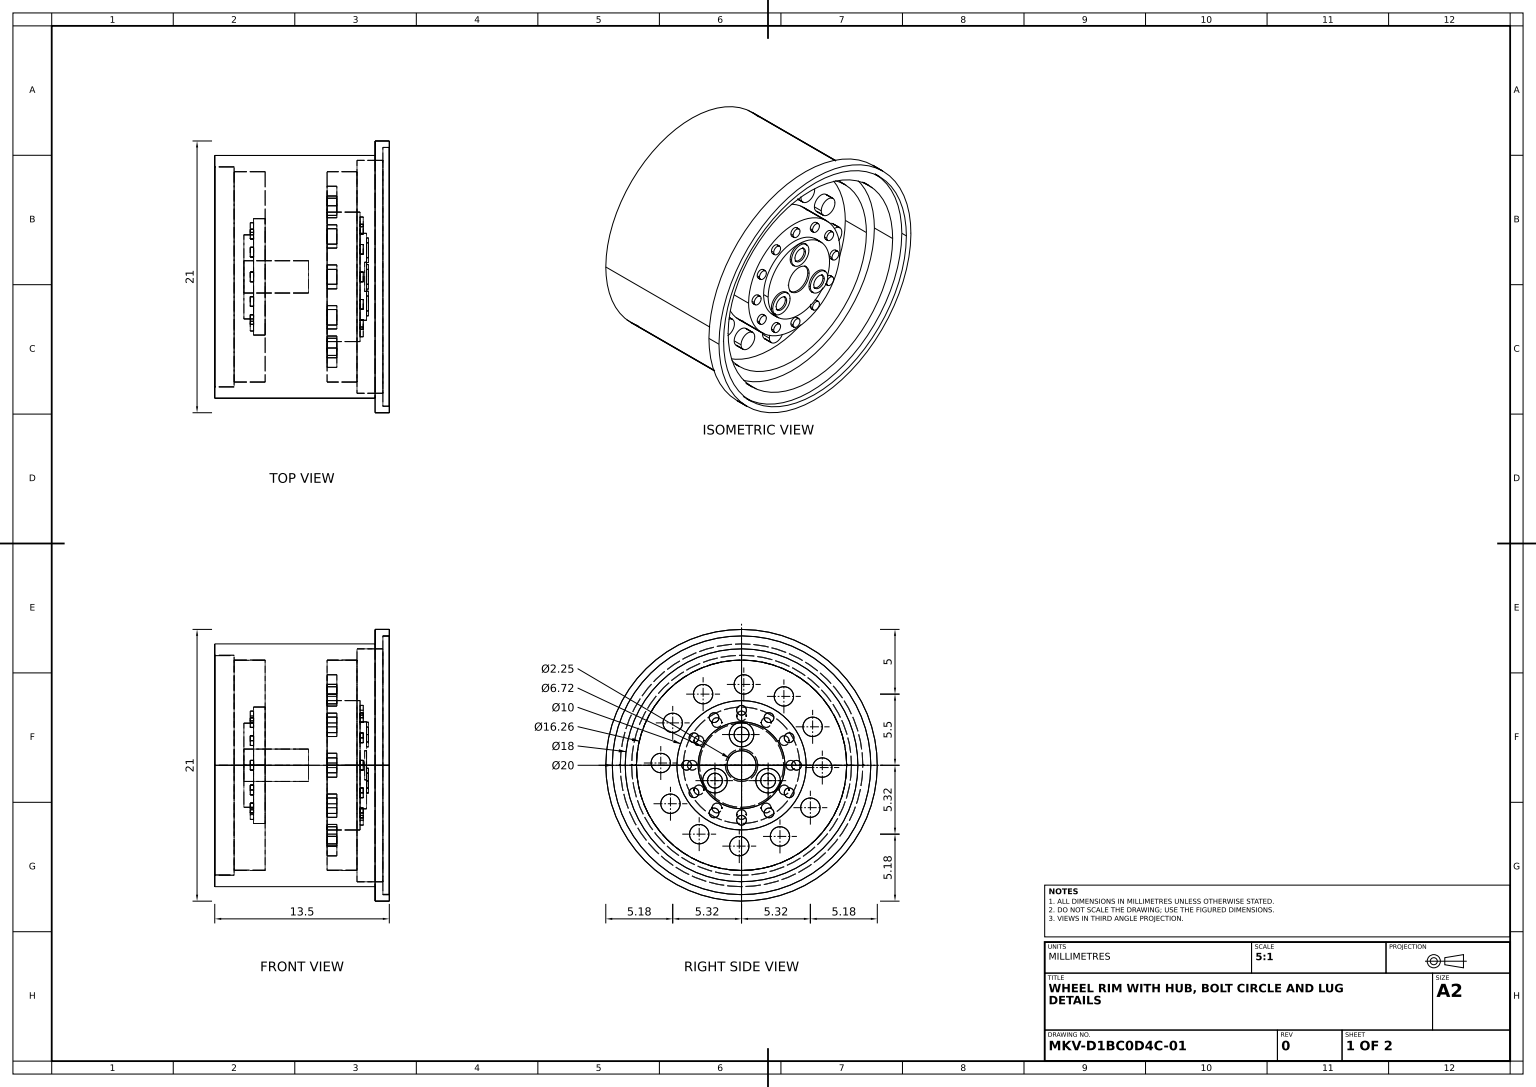
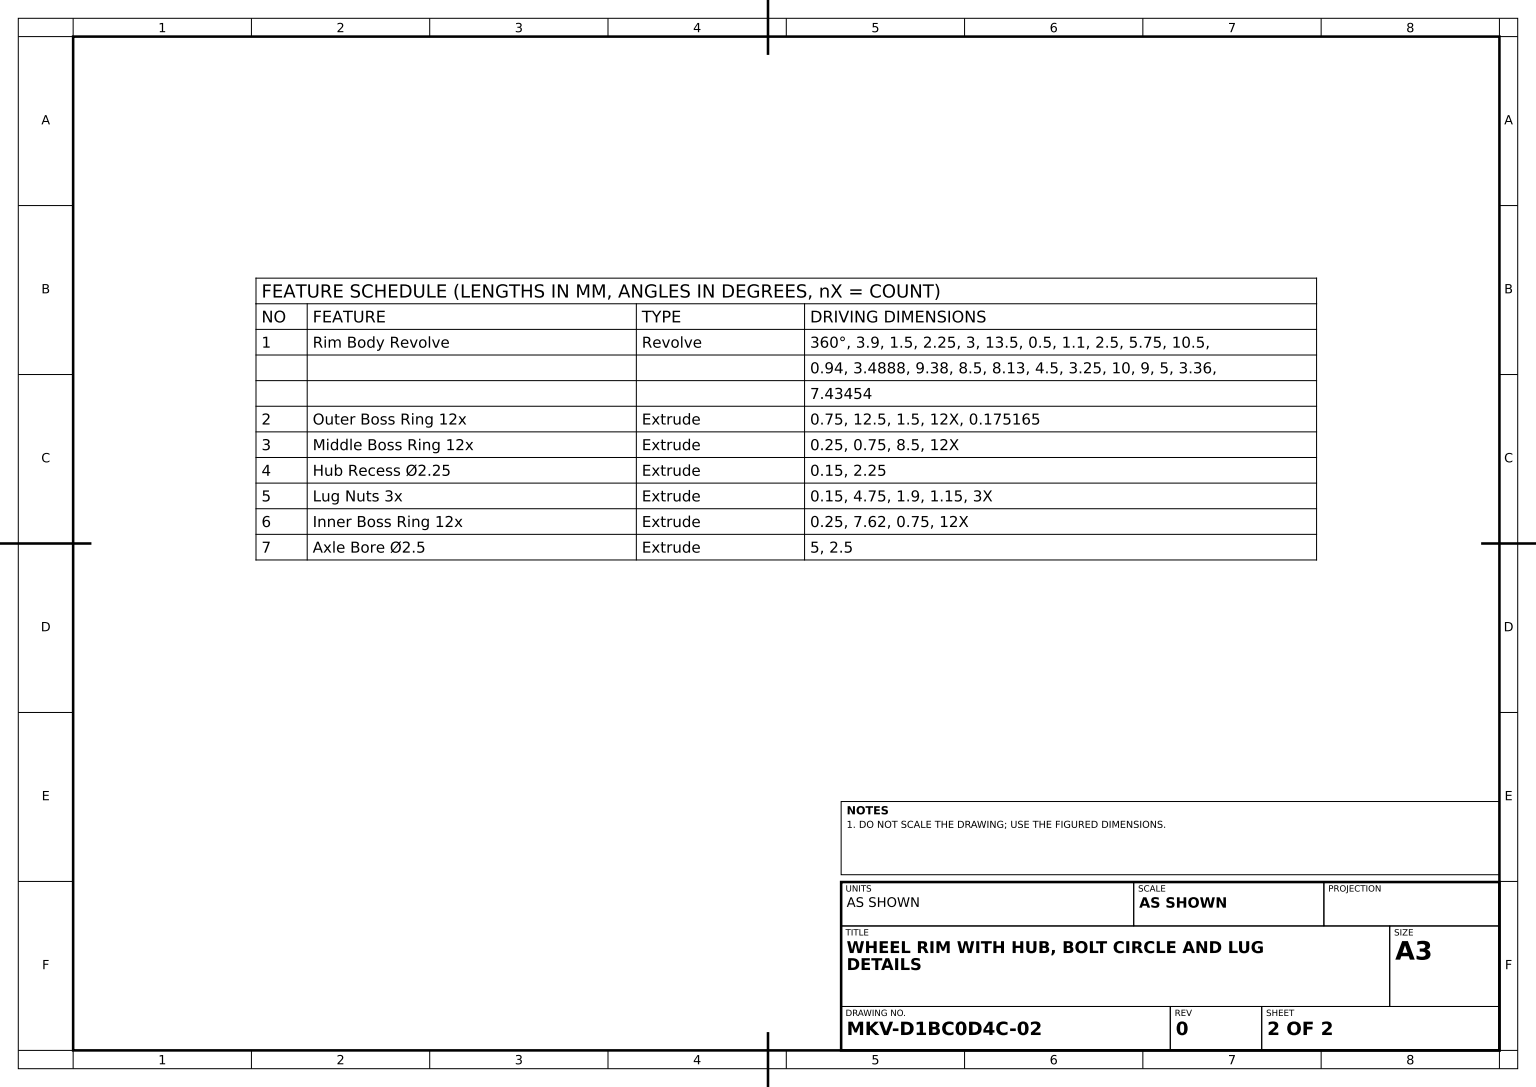
solid
v1 (1.69,6.247545,-0.925165)
v2 (0.94,6.247545,-0.925165)
e1 v1 v2 LINE
v3 (0.94,6.247545,0.574835)
e2 v2 v3 CIRCLE(AX(P(0.94,6.247545,-0.175165),D(1,0,0),D(0,0,-1)),0.75)
v4 (1.69,6.247545,0.574835)
e3 v4 v3 LINE
e4 v1 v4 CIRCLE(AX(P(1.69,6.247545,-0.175165),D(1,0,0),D(0,0,-1)),0.75)
face CYL(AX(P(1.69,6.247545,-0.175165),D(-1,0,0),D(0,0,1)),0.75) [e1 e2 -e3 -e4]
v5 (1.69,-0.175165,-6.997545)
v6 (1.69,-0.175165,-5.497545)
e5 v5 v6 CIRCLE(AX(P(1.69,-0.175165,-6.247545),D(1,0,0),D(0,0,-1)),0.75)
e6 v6 v5 CIRCLE(AX(P(1.69,-0.175165,-6.247545),D(1,0,0),D(0,0,-1)),0.75)
face PLANE(AX(P(1.69,-0.175165,-6.247545),D(1,0,0),D(0,0,-1))) [e5 e6]
v7 (-5,-3.81,0.375)
v8 (-4.75,-3.81,0.375)
e7 v7 v8 LINE
v9 (-5,-3.81,-0.375)
e8 v9 v7 CIRCLE(AX(P(-5,-3.81,0),D(-1,0,0),D(0,0,1)),0.375)
v10 (-4.75,-3.81,-0.375)
e9 v9 v10 LINE
e10 v10 v8 CIRCLE(AX(P(-4.75,-3.81,0),D(-1,0,0),D(0,0,-1)),0.375)
face CYL(AX(P(-5,-3.81,0),D(1,0,0),D(0,0,-1)),0.375) [-e7 -e8 e9 e10]
v11 (1.69,-5.498115,-2.222075)
v12 (1.69,-5.498115,-3.722075)
e11 v11 v12 CIRCLE(AX(P(1.69,-5.498115,-2.972075),D(1,0,0),D(0,0,-1)),0.75)
v13 (0.94,-5.498115,-2.222075)
e12 v11 v13 LINE
v14 (0.94,-5.498115,-3.722075)
e13 v13 v14 CIRCLE(AX(P(0.94,-5.498115,-2.972075),D(1,0,0),D(0,0,-1)),0.75)
e14 v12 v14 LINE
face CYL(AX(P(1.69,-5.498115,-2.972075),D(-1,0,0),D(0,0,1)),0.75) [-e11 e12 e13 -e14]
v15 (1.69,5.32295,-4.02547)
v16 (1.69,5.32295,-2.52547)
e15 v15 v16 CIRCLE(AX(P(1.69,5.32295,-3.27547),D(1,0,0),D(0,0,-1)),0.75)
v17 (0.94,5.32295,-4.02547)
e16 v15 v17 LINE
v18 (0.94,5.32295,-2.52547)
e17 v17 v18 CIRCLE(AX(P(0.94,5.32295,-3.27547),D(1,0,0),D(0,0,-1)),0.75)
e18 v16 v18 LINE
face CYL(AX(P(1.69,5.32295,-3.27547),D(-1,0,0),D(0,0,1)),0.75) [-e15 e16 e17 -e18]
v19 (1.69,2.972075,-6.248115)
v20 (0.94,2.972075,-6.248115)
e19 v19 v20 LINE
v21 (1.69,2.972075,-4.748115)
e20 v21 v19 CIRCLE(AX(P(1.69,2.972075,-5.498115),D(1,0,0),D(0,0,-1)),0.75)
v22 (0.94,2.972075,-4.748115)
e21 v21 v22 LINE
e22 v22 v20 CIRCLE(AX(P(0.94,2.972075,-5.498115),D(1,0,0),D(0,0,-1)),0.75)
face CYL(AX(P(1.69,2.972075,-5.498115),D(-1,0,0),D(0,0,1)),0.75) [-e19 -e20 e21 e22]
v23 (-5,1.905,-2.924557)
v24 (-5,1.905,-3.674557)
e23 v23 v24 CIRCLE(AX(P(-5,1.905,-3.299557),D(-1,0,0),D(0,0,1)),0.375)
e24 v24 v23 CIRCLE(AX(P(-5,1.905,-3.299557),D(-1,0,0),D(0,0,1)),0.375)
face PLANE(AX(P(-5,1.905,-3.299557),D(-1,0,0),D(0,0,1))) [e23 e24]
v25 (-5,-1.905,-2.924557)
v26 (-5,-1.905,-3.674557)
e25 v25 v26 CIRCLE(AX(P(-5,-1.905,-3.299557),D(-1,0,0),D(0,0,1)),0.375)
e26 v26 v25 CIRCLE(AX(P(-5,-1.905,-3.299557),D(-1,0,0),D(0,0,1)),0.375)
face PLANE(AX(P(-5,-1.905,-3.299557),D(-1,0,0),D(0,0,1))) [e25 e26]
e27 v12 v11 CIRCLE(AX(P(1.69,-5.498115,-2.972075),D(1,0,0),D(0,0,-1)),0.75)
face PLANE(AX(P(1.69,-5.498115,-2.972075),D(1,0,0),D(0,0,-1))) [e27 e11]
v27 (4.1388,-1.1875,-1.10681)
v28 (3.9888,-1.1875,-1.10681)
e28 v27 v28 LINE
v29 (4.1388,-1.1875,-3.00681)
e29 v29 v27 CIRCLE(AX(P(4.1388,-1.1875,-2.05681),D(1,0,0),D(0,0,-1)),0.95)
v30 (3.9888,-1.1875,-3.00681)
e30 v29 v30 LINE
e31 v30 v28 CIRCLE(AX(P(3.9888,-1.1875,-2.05681),D(1,0,0),D(0,0,-1)),0.95)
face CYL(AX(P(4.1388,-1.1875,-2.05681),D(-1,0,0),D(0,0,1)),0.95) [-e28 -e29 e30 e31]
v31 (-5,3.299557,1.53)
v32 (-4.75,3.299557,1.53)
e32 v31 v32 LINE
v33 (-5,3.299557,2.28)
e33 v33 v31 CIRCLE(AX(P(-5,3.299557,1.905),D(-1,0,0),D(0,0,1)),0.375)
v34 (-4.75,3.299557,2.28)
e34 v33 v34 LINE
e35 v34 v32 CIRCLE(AX(P(-4.75,3.299557,1.905),D(-1,0,0),D(0,0,-1)),0.375)
face CYL(AX(P(-5,3.299557,1.905),D(1,0,0),D(0,0,-1)),0.375) [-e32 -e33 e34 e35]
v35 (1.69,-2.972075,4.748115)
v36 (1.69,-2.972075,6.248115)
e36 v35 v36 CIRCLE(AX(P(1.69,-2.972075,5.498115),D(1,0,0),D(0,0,-1)),0.75)
e37 v36 v35 CIRCLE(AX(P(1.69,-2.972075,5.498115),D(1,0,0),D(0,0,-1)),0.75)
face PLANE(AX(P(1.69,-2.972075,5.498115),D(1,0,0),D(0,0,-1))) [e36 e37]
v37 (3.7388,-3.680608,2.5)
v38 (3.7388,-3.680608,1.75)
e38 v37 v38 CIRCLE(AX(P(3.7388,-3.680608,2.125),D(1,0,0),D(0,0,-1)),0.375)
v39 (3.4888,-3.680608,2.5)
e39 v37 v39 LINE
v40 (3.4888,-3.680608,1.75)
e40 v39 v40 CIRCLE(AX(P(3.4888,-3.680608,2.125),D(1,0,0),D(0,0,-1)),0.375)
e41 v38 v40 LINE
face CYL(AX(P(3.7388,-3.680608,2.125),D(-1,0,0),D(0,0,1)),0.375) [-e38 e39 e40 -e41]
v41 (0.94,-2.972075,4.748115)
v42 (0.94,-2.972075,6.248115)
e42 v41 v42 CIRCLE(AX(P(0.94,-2.972075,5.498115),D(1,0,0),D(0,0,-1)),0.75)
e43 v36 v42 LINE
e44 v35 v41 LINE
face CYL(AX(P(1.69,-2.972075,5.498115),D(-1,0,0),D(0,0,1)),0.75) [e42 -e43 -e36 e44]
v43 (4.1388,-1.1875,1.48181)
v44 (3.9888,-1.1875,1.48181)
e45 v43 v44 LINE
v45 (4.1388,-1.1875,2.63181)
e46 v43 v45 CIRCLE(AX(P(4.1388,-1.1875,2.05681),D(1,0,0),D(0,0,-1)),0.575)
v46 (3.9888,-1.1875,2.63181)
e47 v45 v46 LINE
e48 v46 v44 CIRCLE(AX(P(3.9888,-1.1875,2.05681),D(-1,0,0),D(0,0,-1)),0.575)
face CYL(AX(P(4.1388,-1.1875,2.05681),D(-1,0,0),D(0,0,1)),0.575) rev [-e45 e46 e47 e48]
v47 (3.7388,2.125,3.305608)
v48 (3.4888,2.125,3.305608)
e49 v47 v48 LINE
v49 (3.4888,2.125,4.055608)
e50 v48 v49 CIRCLE(AX(P(3.4888,2.125,3.680608),D(1,0,0),D(0,0,-1)),0.375)
v50 (3.7388,2.125,4.055608)
e51 v50 v49 LINE
e52 v47 v50 CIRCLE(AX(P(3.7388,2.125,3.680608),D(1,0,0),D(0,0,-1)),0.375)
face CYL(AX(P(3.7388,2.125,3.680608),D(-1,0,0),D(0,0,1)),0.375) [e49 e50 -e51 -e52]
v51 (-4.75,0,4.5)
v52 (-4.75,0,-4.5)
e53 v51 v52 CIRCLE(AX(P(-4.75,0,0),D(-1,0,0),D(0,0,1)),4.5)
v53 (-3.85,0,4.5)
e54 v53 v51 LINE
v54 (-3.85,0,-4.5)
e55 v53 v54 CIRCLE(AX(P(-3.85,0,0),D(-1,0,0),D(0,0,1)),4.5)
e56 v54 v52 LINE
face CYL(AX(P(0,0,0),D(-1,0,0),D(0,0,1)),4.5) [-e53 -e54 e55 e56]
v55 (-4.75,-3.299557,2.28)
v56 (-4.75,-3.299557,1.53)
e57 v55 v56 CIRCLE(AX(P(-4.75,-3.299557,1.905),D(-1,0,0),D(0,0,-1)),0.375)
v57 (-5,-3.299557,1.53)
e58 v57 v56 LINE
v58 (-5,-3.299557,2.28)
e59 v58 v57 CIRCLE(AX(P(-5,-3.299557,1.905),D(-1,0,0),D(0,0,1)),0.375)
e60 v58 v55 LINE
face CYL(AX(P(-5,-3.299557,1.905),D(1,0,0),D(0,0,-1)),0.375) [e57 -e58 -e59 e60]
v59 (3.7388,-4.25,-0.375)
v60 (3.4888,-4.25,-0.375)
e61 v59 v60 LINE
v61 (3.7388,-4.25,0.375)
e62 v61 v59 CIRCLE(AX(P(3.7388,-4.25,0),D(1,0,0),D(0,0,-1)),0.375)
v62 (3.4888,-4.25,0.375)
e63 v61 v62 LINE
e64 v62 v60 CIRCLE(AX(P(3.4888,-4.25,0),D(1,0,0),D(0,0,-1)),0.375)
face CYL(AX(P(3.7388,-4.25,0),D(-1,0,0),D(0,0,1)),0.375) [-e61 -e62 e63 e64]
e65 v42 v41 CIRCLE(AX(P(0.94,-2.972075,5.498115),D(1,0,0),D(0,0,-1)),0.75)
face CYL(AX(P(1.69,-2.972075,5.498115),D(-1,0,0),D(0,0,1)),0.75) [e43 e65 -e44 -e37]
v63 (3.7388,0,-3.875)
v64 (3.7388,0,-4.625)
e66 v63 v64 CIRCLE(AX(P(3.7388,0,-4.25),D(1,0,0),D(0,0,-1)),0.375)
e67 v64 v63 CIRCLE(AX(P(3.7388,0,-4.25),D(1,0,0),D(0,0,-1)),0.375)
face PLANE(AX(P(3.7388,0,-4.25),D(1,0,0),D(0,0,-1))) [e66 e67]
v65 (3.4888,0,-4.625)
v66 (3.4888,0,-3.875)
e68 v65 v66 CIRCLE(AX(P(3.4888,0,-4.25),D(1,0,0),D(0,0,-1)),0.375)
e69 v63 v66 LINE
e70 v64 v65 LINE
face CYL(AX(P(3.7388,0,-4.25),D(-1,0,0),D(0,0,1)),0.375) [e68 -e69 -e67 e70]
e71 v59 v61 CIRCLE(AX(P(3.7388,-4.25,0),D(1,0,0),D(0,0,-1)),0.375)
face PLANE(AX(P(3.7388,-4.25,0),D(1,0,0),D(0,0,-1))) [e62 e71]
v67 (-5,3.299557,-1.53)
v68 (-5,3.299557,-2.28)
e72 v67 v68 CIRCLE(AX(P(-5,3.299557,-1.905),D(-1,0,0),D(0,0,1)),0.375)
v69 (-4.75,3.299557,-1.53)
e73 v67 v69 LINE
v70 (-4.75,3.299557,-2.28)
e74 v69 v70 CIRCLE(AX(P(-4.75,3.299557,-1.905),D(-1,0,0),D(0,0,-1)),0.375)
e75 v68 v70 LINE
face CYL(AX(P(-5,3.299557,-1.905),D(1,0,0),D(0,0,-1)),0.375) [-e72 e73 e74 -e75]
v71 (-4.75,3.81,0.375)
v72 (-4.75,3.81,-0.375)
e76 v71 v72 CIRCLE(AX(P(-4.75,3.81,0),D(-1,0,0),D(0,0,-1)),0.375)
v73 (-5,3.81,-0.375)
e77 v73 v72 LINE
v74 (-5,3.81,0.375)
e78 v74 v73 CIRCLE(AX(P(-5,3.81,0),D(-1,0,0),D(0,0,1)),0.375)
e79 v74 v71 LINE
face CYL(AX(P(-5,3.81,0),D(1,0,0),D(0,0,-1)),0.375) [e76 -e77 -e78 e79]
v75 (-5,0,4.185)
v76 (-5,0,3.435)
e80 v75 v76 CIRCLE(AX(P(-5,0,3.81),D(-1,0,0),D(0,0,1)),0.375)
v77 (-4.75,0,4.185)
e81 v75 v77 LINE
v78 (-4.75,0,3.435)
e82 v77 v78 CIRCLE(AX(P(-4.75,0,3.81),D(-1,0,0),D(0,0,-1)),0.375)
e83 v76 v78 LINE
face CYL(AX(P(-5,0,3.81),D(1,0,0),D(0,0,-1)),0.375) [-e80 e81 e82 -e83]
v79 (-5,-1.905,2.924557)
v80 (-5,-1.905,3.674557)
e84 v79 v80 CIRCLE(AX(P(-5,-1.905,3.299557),D(-1,0,0),D(0,0,1)),0.375)
e85 v80 v79 CIRCLE(AX(P(-5,-1.905,3.299557),D(-1,0,0),D(0,0,1)),0.375)
face PLANE(AX(P(-5,-1.905,3.299557),D(-1,0,0),D(0,0,1))) [e84 e85]
v81 (1.69,0.175165,5.497545)
v82 (0.94,0.175165,5.497545)
e86 v81 v82 LINE
v83 (1.69,0.175165,6.997545)
e87 v83 v81 CIRCLE(AX(P(1.69,0.175165,6.247545),D(1,0,0),D(0,0,-1)),0.75)
v84 (0.94,0.175165,6.997545)
e88 v83 v84 LINE
e89 v84 v82 CIRCLE(AX(P(0.94,0.175165,6.247545),D(1,0,0),D(0,0,-1)),0.75)
face CYL(AX(P(1.69,0.175165,6.247545),D(-1,0,0),D(0,0,1)),0.75) [-e86 -e87 e88 e89]
e90 v31 v33 CIRCLE(AX(P(-5,3.299557,1.905),D(-1,0,0),D(0,0,1)),0.375)
face PLANE(AX(P(-5,3.299557,1.905),D(-1,0,0),D(0,0,1))) [e90 e33]
v85 (-0.5,0,-1.25)
v86 (-0.5,0,1.25)
e91 v85 v86 CIRCLE(AX(P(-0.5,0,0),D(-1,0,0),D(0,0,1)),1.25)
e92 v86 v85 CIRCLE(AX(P(-0.5,0,0),D(-1,0,0),D(0,0,1)),1.25)
face PLANE(AX(P(-0.5,0,0),D(-1,0,0),D(0,0,1))) [e91 e92]
v87 (3.4888,0,5)
v88 (0.94,0,5)
e93 v87 v88 LINE
v89 (0.94,0,-5)
e94 v89 v88 CIRCLE(AX(P(0.94,0,0),D(-1,0,0),D(0,0,1)),5)
v90 (3.4888,0,-5)
e95 v90 v89 LINE
e96 v90 v87 CIRCLE(AX(P(3.4888,0,0),D(-1,0,0),D(0,0,1)),5)
face CYL(AX(P(0,0,0),D(-1,0,0),D(0,0,1)),5) [e93 -e94 -e95 e96]
v91 (-5,-3.299557,-1.53)
v92 (-5,-3.299557,-2.28)
e97 v91 v92 CIRCLE(AX(P(-5,-3.299557,-1.905),D(-1,0,0),D(0,0,1)),0.375)
e98 v92 v91 CIRCLE(AX(P(-5,-3.299557,-1.905),D(-1,0,0),D(0,0,1)),0.375)
face PLANE(AX(P(-5,-3.299557,-1.905),D(-1,0,0),D(0,0,1))) [e97 e98]
v93 (3.7388,-2.125,4.055608)
v94 (3.7388,-2.125,3.305608)
e99 v93 v94 CIRCLE(AX(P(3.7388,-2.125,3.680608),D(1,0,0),D(0,0,-1)),0.375)
e100 v94 v93 CIRCLE(AX(P(3.7388,-2.125,3.680608),D(1,0,0),D(0,0,-1)),0.375)
face PLANE(AX(P(3.7388,-2.125,3.680608),D(1,0,0),D(0,0,-1))) [e99 e100]
v95 (0.94,0,-8.13)
v96 (0.94,0,8.13)
e101 v95 v96 CIRCLE(AX(P(0.94,0,0),D(-1,0,0),D(0,0,1)),8.13)
v97 (3.25,0,8.13)
e102 v97 v96 LINE
v98 (3.25,0,-8.13)
e103 v98 v97 CIRCLE(AX(P(3.25,0,0),D(-1,0,0),D(0,0,1)),8.13)
e104 v98 v95 LINE
face CYL(AX(P(0,0,0),D(-1,0,0),D(0,0,1)),8.13) rev [e101 -e102 -e103 e104]
e105 v81 v83 CIRCLE(AX(P(1.69,0.175165,6.247545),D(1,0,0),D(0,0,-1)),0.75)
face PLANE(AX(P(1.69,0.175165,6.247545),D(1,0,0),D(0,0,-1))) [e105 e87]
v99 (-7.75,0,9.38)
v100 (-7.75,0,-9.38)
e106 v99 v100 CIRCLE(AX(P(-7.75,0,0),D(-1,0,0),D(0,0,1)),9.38)
e107 v100 v99 CIRCLE(AX(P(-7.75,0,0),D(-1,0,0),D(0,0,1)),9.38)
v101 (-7.75,0,8.5)
v102 (-7.75,0,-8.5)
e108 v101 v102 CIRCLE(AX(P(-7.75,0,0),D(-1,0,0),D(0,0,1)),8.5)
e109 v102 v101 CIRCLE(AX(P(-7.75,0,0),D(-1,0,0),D(0,0,1)),8.5)
face PLANE(AX(P(-7.75,0,0),D(1,0,0),D(0,0,-1))) rev [e106 e107] [-e108 -e109]
v103 (3.9888,-1.1875,-2.63181)
v104 (3.9888,-1.1875,-1.48181)
e110 v103 v104 CIRCLE(AX(P(3.9888,-1.1875,-2.05681),D(-1,0,0),D(0,0,-1)),0.575)
v105 (4.1388,-1.1875,-1.48181)
e111 v105 v104 LINE
v106 (4.1388,-1.1875,-2.63181)
e112 v105 v106 CIRCLE(AX(P(4.1388,-1.1875,-2.05681),D(1,0,0),D(0,0,-1)),0.575)
e113 v106 v103 LINE
face CYL(AX(P(4.1388,-1.1875,-2.05681),D(-1,0,0),D(0,0,1)),0.575) rev [e110 -e111 e112 e113]
e114 v7 v9 CIRCLE(AX(P(-5,-3.81,0),D(-1,0,0),D(0,0,1)),0.375)
face PLANE(AX(P(-5,-3.81,0),D(-1,0,0),D(0,0,1))) [e8 e114]
v107 (1.69,3.27547,4.57295)
v108 (1.69,3.27547,6.07295)
e115 v107 v108 CIRCLE(AX(P(1.69,3.27547,5.32295),D(1,0,0),D(0,0,-1)),0.75)
e116 v108 v107 CIRCLE(AX(P(1.69,3.27547,5.32295),D(1,0,0),D(0,0,-1)),0.75)
face PLANE(AX(P(1.69,3.27547,5.32295),D(1,0,0),D(0,0,-1))) [e115 e116]
v109 (1.69,-6.247545,0.925165)
v110 (0.94,-6.247545,0.925165)
e117 v109 v110 LINE
v111 (1.69,-6.247545,-0.574835)
e118 v111 v109 CIRCLE(AX(P(1.69,-6.247545,0.175165),D(1,0,0),D(0,0,-1)),0.75)
v112 (0.94,-6.247545,-0.574835)
e119 v111 v112 LINE
e120 v112 v110 CIRCLE(AX(P(0.94,-6.247545,0.175165),D(1,0,0),D(0,0,-1)),0.75)
face CYL(AX(P(1.69,-6.247545,0.175165),D(-1,0,0),D(0,0,1)),0.75) [-e117 -e118 e119 e120]
v113 (-4.75,1.905,3.674557)
v114 (-4.75,1.905,2.924557)
e121 v113 v114 CIRCLE(AX(P(-4.75,1.905,3.299557),D(-1,0,0),D(0,0,-1)),0.375)
v115 (-5,1.905,2.924557)
e122 v115 v114 LINE
v116 (-5,1.905,3.674557)
e123 v116 v115 CIRCLE(AX(P(-5,1.905,3.299557),D(-1,0,0),D(0,0,1)),0.375)
e124 v116 v113 LINE
face CYL(AX(P(-5,1.905,3.299557),D(1,0,0),D(0,0,-1)),0.375) [e121 -e122 -e123 e124]
v117 (3.7388,3.680608,1.75)
v118 (3.4888,3.680608,1.75)
e125 v117 v118 LINE
v119 (3.7388,3.680608,2.5)
e126 v119 v117 CIRCLE(AX(P(3.7388,3.680608,2.125),D(1,0,0),D(0,0,-1)),0.375)
v120 (3.4888,3.680608,2.5)
e127 v119 v120 LINE
e128 v120 v118 CIRCLE(AX(P(3.4888,3.680608,2.125),D(1,0,0),D(0,0,-1)),0.375)
face CYL(AX(P(3.7388,3.680608,2.125),D(-1,0,0),D(0,0,1)),0.375) [-e125 -e126 e127 e128]
v121 (4.1388,2.375,0.95)
v122 (4.1388,2.375,-0.95)
e129 v121 v122 CIRCLE(AX(P(4.1388,2.375,0),D(1,0,0),D(0,0,-1)),0.95)
v123 (3.9888,2.375,0.95)
e130 v121 v123 LINE
v124 (3.9888,2.375,-0.95)
e131 v123 v124 CIRCLE(AX(P(3.9888,2.375,0),D(1,0,0),D(0,0,-1)),0.95)
e132 v122 v124 LINE
face CYL(AX(P(4.1388,2.375,0),D(-1,0,0),D(0,0,1)),0.95) [-e129 e130 e131 -e132]
v125 (3.7388,3.680608,-2.5)
v126 (3.4888,3.680608,-2.5)
e133 v125 v126 LINE
v127 (3.7388,3.680608,-1.75)
e134 v127 v125 CIRCLE(AX(P(3.7388,3.680608,-2.125),D(1,0,0),D(0,0,-1)),0.375)
v128 (3.4888,3.680608,-1.75)
e135 v127 v128 LINE
e136 v128 v126 CIRCLE(AX(P(3.4888,3.680608,-2.125),D(1,0,0),D(0,0,-1)),0.375)
face CYL(AX(P(3.7388,3.680608,-2.125),D(-1,0,0),D(0,0,1)),0.375) [-e133 -e134 e135 e136]
v129 (3.9888,0,1.125)
v130 (3.9888,0,-1.125)
e137 v129 v130 CIRCLE(AX(P(3.9888,0,0),D(1,0,0),D(0,0,-1)),1.125)
v131 (3.8388,0,-1.125)
e138 v131 v130 LINE
v132 (3.8388,0,1.125)
e139 v132 v131 CIRCLE(AX(P(3.8388,0,0),D(1,0,0),D(0,0,-1)),1.125)
e140 v132 v129 LINE
face CYL(AX(P(3.8388,0,0),D(1,0,0),D(0,0,-1)),1.125) rev [e137 -e138 -e139 e140]
v133 (3.7388,-2.125,-4.055608)
v134 (3.7388,-2.125,-3.305608)
e141 v133 v134 CIRCLE(AX(P(3.7388,-2.125,-3.680608),D(1,0,0),D(0,0,-1)),0.375)
e142 v134 v133 CIRCLE(AX(P(3.7388,-2.125,-3.680608),D(1,0,0),D(0,0,-1)),0.375)
face PLANE(AX(P(3.7388,-2.125,-3.680608),D(1,0,0),D(0,0,-1))) [e141 e142]
e143 v44 v46 CIRCLE(AX(P(3.9888,-1.1875,2.05681),D(-1,0,0),D(0,0,-1)),0.575)
e144 v45 v43 CIRCLE(AX(P(4.1388,-1.1875,2.05681),D(1,0,0),D(0,0,-1)),0.575)
face CYL(AX(P(4.1388,-1.1875,2.05681),D(-1,0,0),D(0,0,1)),0.575) rev [e45 e143 -e47 e144]
v135 (-4.75,1.905,-3.674557)
e145 v24 v135 LINE
v136 (-4.75,1.905,-2.924557)
e146 v135 v136 CIRCLE(AX(P(-4.75,1.905,-3.299557),D(-1,0,0),D(0,0,-1)),0.375)
e147 v23 v136 LINE
face CYL(AX(P(-5,1.905,-3.299557),D(1,0,0),D(0,0,-1)),0.375) [-e24 e145 e146 -e147]
v137 (0.94,3.27547,4.57295)
v138 (0.94,3.27547,6.07295)
e148 v137 v138 CIRCLE(AX(P(0.94,3.27547,5.32295),D(1,0,0),D(0,0,-1)),0.75)
e149 v138 v137 CIRCLE(AX(P(0.94,3.27547,5.32295),D(1,0,0),D(0,0,-1)),0.75)
v139 (0.94,-0.175165,-5.497545)
v140 (0.94,-0.175165,-6.997545)
e150 v139 v140 CIRCLE(AX(P(0.94,-0.175165,-6.247545),D(1,0,0),D(0,0,-1)),0.75)
e151 v140 v139 CIRCLE(AX(P(0.94,-0.175165,-6.247545),D(1,0,0),D(0,0,-1)),0.75)
e152 v20 v22 CIRCLE(AX(P(0.94,2.972075,-5.498115),D(1,0,0),D(0,0,-1)),0.75)
e153 v96 v95 CIRCLE(AX(P(0.94,0,0),D(-1,0,0),D(0,0,1)),8.13)
v141 (0.94,5.498115,3.722075)
v142 (0.94,5.498115,2.222075)
e154 v141 v142 CIRCLE(AX(P(0.94,5.498115,2.972075),D(1,0,0),D(0,0,-1)),0.75)
e155 v142 v141 CIRCLE(AX(P(0.94,5.498115,2.972075),D(1,0,0),D(0,0,-1)),0.75)
v143 (0.94,-5.32295,2.52547)
v144 (0.94,-5.32295,4.02547)
e156 v143 v144 CIRCLE(AX(P(0.94,-5.32295,3.27547),D(1,0,0),D(0,0,-1)),0.75)
e157 v144 v143 CIRCLE(AX(P(0.94,-5.32295,3.27547),D(1,0,0),D(0,0,-1)),0.75)
v145 (0.94,-3.27547,-6.07295)
v146 (0.94,-3.27547,-4.57295)
e158 v145 v146 CIRCLE(AX(P(0.94,-3.27547,-5.32295),D(1,0,0),D(0,0,-1)),0.75)
e159 v146 v145 CIRCLE(AX(P(0.94,-3.27547,-5.32295),D(1,0,0),D(0,0,-1)),0.75)
e160 v18 v17 CIRCLE(AX(P(0.94,5.32295,-3.27547),D(1,0,0),D(0,0,-1)),0.75)
e161 v3 v2 CIRCLE(AX(P(0.94,6.247545,-0.175165),D(1,0,0),D(0,0,-1)),0.75)
e162 v14 v13 CIRCLE(AX(P(0.94,-5.498115,-2.972075),D(1,0,0),D(0,0,-1)),0.75)
e163 v82 v84 CIRCLE(AX(P(0.94,0.175165,6.247545),D(1,0,0),D(0,0,-1)),0.75)
e164 v88 v89 CIRCLE(AX(P(0.94,0,0),D(-1,0,0),D(0,0,1)),5)
e165 v110 v112 CIRCLE(AX(P(0.94,-6.247545,0.175165),D(1,0,0),D(0,0,-1)),0.75)
face PLANE(AX(P(0.94,0,0),D(1,0,0),D(0,0,-1))) [-e148 -e149] [-e150 -e151] [-e152 -e22] [-e101 -e153] [-e154 -e155] [-e156 -e157] [-e158 -e159] [-e65 -e42] [-e160 -e17] [-e2 -e161] [-e162 -e13] [-e163 -e89] [e164 e94] [-e165 -e120]
e166 v130 v129 CIRCLE(AX(P(3.9888,0,0),D(1,0,0),D(0,0,-1)),1.125)
e167 v131 v132 CIRCLE(AX(P(3.8388,0,0),D(1,0,0),D(0,0,-1)),1.125)
face CYL(AX(P(3.8388,0,0),D(1,0,0),D(0,0,-1)),1.125) rev [e138 e166 -e140 -e167]
v147 (5.75,0,10.5)
v148 (4.65,0,10.5)
e168 v147 v148 LINE
v149 (5.75,0,-10.5)
e169 v147 v149 CIRCLE(AX(P(5.75,0,0),D(-1,0,0),D(0,0,1)),10.5)
v150 (4.65,0,-10.5)
e170 v149 v150 LINE
e171 v148 v150 CIRCLE(AX(P(4.65,0,0),D(-1,0,0),D(0,0,1)),10.5)
face CYL(AX(P(0,0,0),D(-1,0,0),D(0,0,1)),10.5) [-e168 e169 e170 -e171]
e172 v28 v30 CIRCLE(AX(P(3.9888,-1.1875,-2.05681),D(1,0,0),D(0,0,-1)),0.95)
e173 v124 v123 CIRCLE(AX(P(3.9888,2.375,0),D(1,0,0),D(0,0,-1)),0.95)
v151 (3.9888,0,-3.36)
v152 (3.9888,0,3.36)
e174 v151 v152 CIRCLE(AX(P(3.9888,0,0),D(-1,0,0),D(0,0,1)),3.36)
e175 v152 v151 CIRCLE(AX(P(3.9888,0,0),D(-1,0,0),D(0,0,1)),3.36)
v153 (3.9888,-1.1875,3.00681)
v154 (3.9888,-1.1875,1.10681)
e176 v153 v154 CIRCLE(AX(P(3.9888,-1.1875,2.05681),D(1,0,0),D(0,0,-1)),0.95)
e177 v154 v153 CIRCLE(AX(P(3.9888,-1.1875,2.05681),D(1,0,0),D(0,0,-1)),0.95)
face PLANE(AX(P(3.9888,0,0),D(1,0,0),D(0,0,-1))) [-e31 -e172] [-e166 -e137] [-e131 -e173] [-e174 -e175] [-e176 -e177]
v155 (-5,0,-3.435)
v156 (-5,0,-4.185)
e178 v155 v156 CIRCLE(AX(P(-5,0,-3.81),D(-1,0,0),D(0,0,1)),0.375)
e179 v156 v155 CIRCLE(AX(P(-5,0,-3.81),D(-1,0,0),D(0,0,1)),0.375)
face PLANE(AX(P(-5,0,-3.81),D(-1,0,0),D(0,0,1))) [e178 e179]
e180 v72 v71 CIRCLE(AX(P(-4.75,3.81,0),D(-1,0,0),D(0,0,-1)),0.375)
e181 v73 v74 CIRCLE(AX(P(-5,3.81,0),D(-1,0,0),D(0,0,1)),0.375)
face CYL(AX(P(-5,3.81,0),D(1,0,0),D(0,0,-1)),0.375) [e180 -e79 -e181 e77]
v157 (4.1388,2.375,0.575)
v158 (4.1388,2.375,-0.575)
e182 v157 v158 CIRCLE(AX(P(4.1388,2.375,0),D(1,0,0),D(0,0,-1)),0.575)
e183 v158 v157 CIRCLE(AX(P(4.1388,2.375,0),D(1,0,0),D(0,0,-1)),0.575)
e184 v122 v121 CIRCLE(AX(P(4.1388,2.375,0),D(1,0,0),D(0,0,-1)),0.95)
face PLANE(AX(P(4.1388,2.375,0),D(1,0,0),D(0,0,-1))) [-e182 -e183] [e184 e129]
v159 (3.4888,-2.125,4.055608)
e185 v93 v159 LINE
v160 (3.4888,-2.125,3.305608)
e186 v159 v160 CIRCLE(AX(P(3.4888,-2.125,3.680608),D(1,0,0),D(0,0,-1)),0.375)
e187 v94 v160 LINE
face CYL(AX(P(3.7388,-2.125,3.680608),D(-1,0,0),D(0,0,1)),0.375) [-e99 e185 e186 -e187]
v161 (-3.85,0,-8.13)
v162 (-6.25,0,-8.13)
e188 v161 v162 LINE
v163 (-6.25,0,8.13)
e189 v162 v163 CIRCLE(AX(P(-6.25,0,0),D(-1,0,0),D(0,0,1)),8.13)
v164 (-3.85,0,8.13)
e190 v164 v163 LINE
e191 v161 v164 CIRCLE(AX(P(-3.85,0,0),D(-1,0,0),D(0,0,1)),8.13)
face CYL(AX(P(0,0,0),D(-1,0,0),D(0,0,1)),8.13) rev [e188 e189 -e190 -e191]
face CYL(AX(P(4.1388,2.375,0),D(-1,0,0),D(0,0,1)),0.95) [-e130 -e184 e132 e173]
v165 (1.69,-3.27547,-6.07295)
e192 v165 v145 LINE
v166 (1.69,-3.27547,-4.57295)
e193 v166 v165 CIRCLE(AX(P(1.69,-3.27547,-5.32295),D(1,0,0),D(0,0,-1)),0.75)
e194 v166 v146 LINE
face CYL(AX(P(1.69,-3.27547,-5.32295),D(-1,0,0),D(0,0,1)),0.75) [e159 -e192 -e193 e194]
v167 (5.75,0,-10)
v168 (5.75,0,10)
e195 v167 v168 CIRCLE(AX(P(5.75,0,0),D(-1,0,0),D(0,0,1)),10)
e196 v168 v167 CIRCLE(AX(P(5.75,0,0),D(-1,0,0),D(0,0,1)),10)
e197 v149 v147 CIRCLE(AX(P(5.75,0,0),D(-1,0,0),D(0,0,1)),10.5)
face PLANE(AX(P(5.75,0,0),D(1,0,0),D(0,0,-1))) [e195 e196] [-e197 -e169]
e198 v70 v69 CIRCLE(AX(P(-4.75,3.299557,-1.905),D(-1,0,0),D(0,0,-1)),0.375)
e199 v68 v67 CIRCLE(AX(P(-5,3.299557,-1.905),D(-1,0,0),D(0,0,1)),0.375)
face CYL(AX(P(-5,3.299557,-1.905),D(1,0,0),D(0,0,-1)),0.375) [e198 -e73 -e199 e75]
v169 (5.25,0,10)
e200 v168 v169 LINE
v170 (5.25,0,-10)
e201 v169 v170 CIRCLE(AX(P(5.25,0,0),D(-1,0,0),D(0,0,1)),10)
e202 v167 v170 LINE
face CYL(AX(P(0,0,0),D(-1,0,0),D(0,0,1)),10) rev [-e196 e200 e201 -e202]
v171 (3.4888,2.125,-3.305608)
v172 (3.4888,2.125,-4.055608)
e203 v171 v172 CIRCLE(AX(P(3.4888,2.125,-3.680608),D(1,0,0),D(0,0,-1)),0.375)
v173 (3.7388,2.125,-4.055608)
e204 v173 v172 LINE
v174 (3.7388,2.125,-3.305608)
e205 v174 v173 CIRCLE(AX(P(3.7388,2.125,-3.680608),D(1,0,0),D(0,0,-1)),0.375)
e206 v174 v171 LINE
face CYL(AX(P(3.7388,2.125,-3.680608),D(-1,0,0),D(0,0,1)),0.375) [e203 -e204 -e205 e206]
e207 v104 v103 CIRCLE(AX(P(3.9888,-1.1875,-2.05681),D(-1,0,0),D(0,0,-1)),0.575)
face PLANE(AX(P(3.9888,0,0),D(1,0,0),D(0,0,-1))) [-e207 -e110]
v175 (-5.5,0,-3.25)
v176 (-5.5,0,3.25)
e208 v175 v176 CIRCLE(AX(P(-5.5,0,0),D(-1,0,0),D(0,0,1)),3.25)
e209 v176 v175 CIRCLE(AX(P(-5.5,0,0),D(-1,0,0),D(0,0,1)),3.25)
v177 (-5.5,0,-1.25)
v178 (-5.5,0,1.25)
e210 v177 v178 CIRCLE(AX(P(-5.5,0,0),D(-1,0,0),D(0,0,1)),1.25)
e211 v178 v177 CIRCLE(AX(P(-5.5,0,0),D(-1,0,0),D(0,0,1)),1.25)
face PLANE(AX(P(-5.5,0,0),D(1,0,0),D(0,0,-1))) rev [e208 e209] [-e210 -e211]
e212 v117 v119 CIRCLE(AX(P(3.7388,3.680608,2.125),D(1,0,0),D(0,0,-1)),0.375)
face PLANE(AX(P(3.7388,3.680608,2.125),D(1,0,0),D(0,0,-1))) [e126 e212]
v179 (-4.75,-3.299557,-2.28)
e213 v92 v179 LINE
v180 (-4.75,-3.299557,-1.53)
e214 v179 v180 CIRCLE(AX(P(-4.75,-3.299557,-1.905),D(-1,0,0),D(0,0,-1)),0.375)
e215 v91 v180 LINE
face CYL(AX(P(-5,-3.299557,-1.905),D(1,0,0),D(0,0,-1)),0.375) [-e98 e213 e214 -e215]
v181 (3.7388,0,4.625)
v182 (3.7388,0,3.875)
e216 v181 v182 CIRCLE(AX(P(3.7388,0,4.25),D(1,0,0),D(0,0,-1)),0.375)
e217 v182 v181 CIRCLE(AX(P(3.7388,0,4.25),D(1,0,0),D(0,0,-1)),0.375)
face PLANE(AX(P(3.7388,0,4.25),D(1,0,0),D(0,0,-1))) [e216 e217]
v183 (3.7388,4.25,-0.375)
v184 (3.7388,4.25,0.375)
e218 v183 v184 CIRCLE(AX(P(3.7388,4.25,0),D(1,0,0),D(0,0,-1)),0.375)
e219 v184 v183 CIRCLE(AX(P(3.7388,4.25,0),D(1,0,0),D(0,0,-1)),0.375)
face PLANE(AX(P(3.7388,4.25,0),D(1,0,0),D(0,0,-1))) [e218 e219]
face PLANE(AX(P(-5,3.81,0),D(-1,0,0),D(0,0,1))) [e181 e78]
e220 v54 v53 CIRCLE(AX(P(-3.85,0,0),D(-1,0,0),D(0,0,1)),4.5)
e221 v52 v51 CIRCLE(AX(P(-4.75,0,0),D(-1,0,0),D(0,0,1)),4.5)
face CYL(AX(P(0,0,0),D(-1,0,0),D(0,0,1)),4.5) [-e56 e220 e54 -e221]
v185 (-4.75,0,-3.435)
e222 v155 v185 LINE
v186 (-4.75,0,-4.185)
e223 v185 v186 CIRCLE(AX(P(-4.75,0,-3.81),D(-1,0,0),D(0,0,-1)),0.375)
e224 v156 v186 LINE
face CYL(AX(P(-5,0,-3.81),D(1,0,0),D(0,0,-1)),0.375) [-e178 e222 e223 -e224]
e225 v118 v120 CIRCLE(AX(P(3.4888,3.680608,2.125),D(1,0,0),D(0,0,-1)),0.375)
face CYL(AX(P(3.7388,3.680608,2.125),D(-1,0,0),D(0,0,1)),0.375) [-e212 e125 e225 -e127]
v187 (3.4888,0,3.36)
e226 v152 v187 LINE
v188 (3.4888,0,-3.36)
e227 v188 v187 CIRCLE(AX(P(3.4888,0,0),D(-1,0,0),D(0,0,1)),3.36)
e228 v151 v188 LINE
face CYL(AX(P(0,0,0),D(-1,0,0),D(0,0,1)),3.36) [e174 e226 -e227 -e228]
v189 (3.9888,2.375,0.575)
v190 (3.9888,2.375,-0.575)
e229 v189 v190 CIRCLE(AX(P(3.9888,2.375,0),D(-1,0,0),D(0,0,-1)),0.575)
e230 v190 v189 CIRCLE(AX(P(3.9888,2.375,0),D(-1,0,0),D(0,0,-1)),0.575)
face PLANE(AX(P(3.9888,0,0),D(1,0,0),D(0,0,-1))) [-e229 -e230]
v191 (3.7388,-3.680608,-1.75)
v192 (3.7388,-3.680608,-2.5)
e231 v191 v192 CIRCLE(AX(P(3.7388,-3.680608,-2.125),D(1,0,0),D(0,0,-1)),0.375)
e232 v192 v191 CIRCLE(AX(P(3.7388,-3.680608,-2.125),D(1,0,0),D(0,0,-1)),0.375)
face PLANE(AX(P(3.7388,-3.680608,-2.125),D(1,0,0),D(0,0,-1))) [e231 e232]
v193 (3.4888,0,3.875)
e233 v182 v193 LINE
v194 (3.4888,0,4.625)
e234 v193 v194 CIRCLE(AX(P(3.4888,0,4.25),D(1,0,0),D(0,0,-1)),0.375)
e235 v181 v194 LINE
face CYL(AX(P(3.7388,0,4.25),D(-1,0,0),D(0,0,1)),0.375) [-e217 e233 e234 -e235]
v195 (3.4888,4.25,0.375)
e236 v184 v195 LINE
v196 (3.4888,4.25,-0.375)
e237 v195 v196 CIRCLE(AX(P(3.4888,4.25,0),D(1,0,0),D(0,0,-1)),0.375)
e238 v183 v196 LINE
face CYL(AX(P(3.7388,4.25,0),D(-1,0,0),D(0,0,1)),0.375) [-e219 e236 e237 -e238]
e239 v164 v161 CIRCLE(AX(P(-3.85,0,0),D(-1,0,0),D(0,0,1)),8.13)
e240 v163 v162 CIRCLE(AX(P(-6.25,0,0),D(-1,0,0),D(0,0,1)),8.13)
face CYL(AX(P(0,0,0),D(-1,0,0),D(0,0,1)),8.13) rev [-e188 -e239 e190 e240]
e241 v5 v140 LINE
e242 v6 v139 LINE
face CYL(AX(P(1.69,-0.175165,-6.247545),D(-1,0,0),D(0,0,1)),0.75) [e150 -e241 -e6 e242]
v197 (1.69,5.498115,2.222075)
e243 v197 v142 LINE
v198 (1.69,5.498115,3.722075)
e244 v198 v197 CIRCLE(AX(P(1.69,5.498115,2.972075),D(1,0,0),D(0,0,-1)),0.75)
e245 v198 v141 LINE
face CYL(AX(P(1.69,5.498115,2.972075),D(-1,0,0),D(0,0,1)),0.75) [e154 -e243 -e244 e245]
e246 v76 v75 CIRCLE(AX(P(-5,0,3.81),D(-1,0,0),D(0,0,1)),0.375)
face PLANE(AX(P(-5,0,3.81),D(-1,0,0),D(0,0,1))) [e246 e80]
e247 v125 v127 CIRCLE(AX(P(3.7388,3.680608,-2.125),D(1,0,0),D(0,0,-1)),0.375)
face PLANE(AX(P(3.7388,3.680608,-2.125),D(1,0,0),D(0,0,-1))) [e247 e134]
e248 v106 v105 CIRCLE(AX(P(4.1388,-1.1875,-2.05681),D(1,0,0),D(0,0,-1)),0.575)
e249 v27 v29 CIRCLE(AX(P(4.1388,-1.1875,-2.05681),D(1,0,0),D(0,0,-1)),0.95)
face PLANE(AX(P(4.1388,-1.1875,-2.05681),D(1,0,0),D(0,0,-1))) [-e112 -e248] [e249 e29]
v199 (4.1388,-1.1875,1.10681)
e250 v199 v154 LINE
v200 (4.1388,-1.1875,3.00681)
e251 v200 v199 CIRCLE(AX(P(4.1388,-1.1875,2.05681),D(1,0,0),D(0,0,-1)),0.95)
e252 v200 v153 LINE
face CYL(AX(P(4.1388,-1.1875,2.05681),D(-1,0,0),D(0,0,1)),0.95) [e176 -e250 -e251 e252]
e253 v32 v34 CIRCLE(AX(P(-4.75,3.299557,1.905),D(-1,0,0),D(0,0,-1)),0.375)
face CYL(AX(P(-5,3.299557,1.905),D(1,0,0),D(0,0,-1)),0.375) [-e34 -e90 e32 e253]
e254 v187 v188 CIRCLE(AX(P(3.4888,0,0),D(-1,0,0),D(0,0,1)),3.36)
face CYL(AX(P(0,0,0),D(-1,0,0),D(0,0,1)),3.36) [e228 -e254 -e226 e175]
e255 v172 v171 CIRCLE(AX(P(3.4888,2.125,-3.680608),D(1,0,0),D(0,0,-1)),0.375)
e256 v173 v174 CIRCLE(AX(P(3.7388,2.125,-3.680608),D(1,0,0),D(0,0,-1)),0.375)
face CYL(AX(P(3.7388,2.125,-3.680608),D(-1,0,0),D(0,0,1)),0.375) [e204 e255 -e206 -e256]
e257 v86 v178 LINE
e258 v85 v177 LINE
face CYL(AX(P(-0.5,0,0),D(-1,0,0),D(0,0,1)),1.25) rev [-e92 e257 e211 -e258]
face PLANE(AX(P(3.9888,0,0),D(1,0,0),D(0,0,-1))) [-e143 -e48]
face CYL(AX(P(1.69,-5.498115,-2.972075),D(-1,0,0),D(0,0,1)),0.75) [-e27 e14 e162 -e12]
e259 v60 v62 CIRCLE(AX(P(3.4888,-4.25,0),D(1,0,0),D(0,0,-1)),0.375)
face CYL(AX(P(3.7388,-4.25,0),D(-1,0,0),D(0,0,1)),0.375) [-e63 -e71 e61 e259]
v201 (-4.75,-1.905,-2.924557)
e260 v25 v201 LINE
v202 (-4.75,-1.905,-3.674557)
e261 v201 v202 CIRCLE(AX(P(-4.75,-1.905,-3.299557),D(-1,0,0),D(0,0,-1)),0.375)
e262 v26 v202 LINE
face CYL(AX(P(-5,-1.905,-3.299557),D(1,0,0),D(0,0,-1)),0.375) [-e25 e260 e261 -e262]
e263 v66 v65 CIRCLE(AX(P(3.4888,0,-4.25),D(1,0,0),D(0,0,-1)),0.375)
face CYL(AX(P(3.7388,0,-4.25),D(-1,0,0),D(0,0,1)),0.375) [-e66 e69 e263 -e70]
e264 v8 v10 CIRCLE(AX(P(-4.75,-3.81,0),D(-1,0,0),D(0,0,-1)),0.375)
face CYL(AX(P(-5,-3.81,0),D(1,0,0),D(0,0,-1)),0.375) [e264 -e9 -e114 e7]
v203 (3.4888,-3.680608,-2.5)
v204 (3.4888,-3.680608,-1.75)
e265 v203 v204 CIRCLE(AX(P(3.4888,-3.680608,-2.125),D(1,0,0),D(0,0,-1)),0.375)
e266 v204 v203 CIRCLE(AX(P(3.4888,-3.680608,-2.125),D(1,0,0),D(0,0,-1)),0.375)
e267 v40 v39 CIRCLE(AX(P(3.4888,-3.680608,2.125),D(1,0,0),D(0,0,-1)),0.375)
v205 (3.4888,-2.125,-3.305608)
v206 (3.4888,-2.125,-4.055608)
e268 v205 v206 CIRCLE(AX(P(3.4888,-2.125,-3.680608),D(1,0,0),D(0,0,-1)),0.375)
e269 v206 v205 CIRCLE(AX(P(3.4888,-2.125,-3.680608),D(1,0,0),D(0,0,-1)),0.375)
e270 v160 v159 CIRCLE(AX(P(3.4888,-2.125,3.680608),D(1,0,0),D(0,0,-1)),0.375)
e271 v194 v193 CIRCLE(AX(P(3.4888,0,4.25),D(1,0,0),D(0,0,-1)),0.375)
e272 v126 v128 CIRCLE(AX(P(3.4888,3.680608,-2.125),D(1,0,0),D(0,0,-1)),0.375)
e273 v196 v195 CIRCLE(AX(P(3.4888,4.25,0),D(1,0,0),D(0,0,-1)),0.375)
e274 v87 v90 CIRCLE(AX(P(3.4888,0,0),D(-1,0,0),D(0,0,1)),5)
e275 v49 v48 CIRCLE(AX(P(3.4888,2.125,3.680608),D(1,0,0),D(0,0,-1)),0.375)
face PLANE(AX(P(3.4888,0,0),D(1,0,0),D(0,0,-1))) [-e265 -e266] [-e259 -e64] [-e40 -e267] [-e268 -e269] [-e186 -e270] [e227 e254] [-e234 -e271] [-e272 -e136] [-e237 -e273] [-e263 -e68] [-e255 -e203] [-e96 -e274] [-e128 -e225] [-e275 -e50]
e276 v165 v166 CIRCLE(AX(P(1.69,-3.27547,-5.32295),D(1,0,0),D(0,0,-1)),0.75)
face PLANE(AX(P(1.69,-3.27547,-5.32295),D(1,0,0),D(0,0,-1))) [e276 e193]
v207 (4.65,0,9.38)
v208 (4.65,0,-9.38)
e277 v207 v208 CIRCLE(AX(P(4.65,0,0),D(-1,0,0),D(0,0,1)),9.38)
e278 v208 v207 CIRCLE(AX(P(4.65,0,0),D(-1,0,0),D(0,0,1)),9.38)
e279 v150 v148 CIRCLE(AX(P(4.65,0,0),D(-1,0,0),D(0,0,1)),10.5)
face PLANE(AX(P(4.65,0,0),D(-1,0,0),D(0,0,1))) [-e277 -e278] [e171 e279]
e280 v97 v98 CIRCLE(AX(P(3.25,0,0),D(-1,0,0),D(0,0,1)),8.13)
face CYL(AX(P(0,0,0),D(-1,0,0),D(0,0,1)),8.13) rev [e102 e153 -e104 -e280]
face PLANE(AX(P(3.8388,0,0),D(1,0,0),D(0,0,-1))) [e139 e167]
v209 (5.25,0,9)
v210 (3.25,0,9)
e281 v209 v210 LINE
v211 (3.25,0,-9)
e282 v210 v211 CIRCLE(AX(P(3.25,0,0),D(-1,0,0),D(0,0,1)),9)
v212 (5.25,0,-9)
e283 v212 v211 LINE
e284 v209 v212 CIRCLE(AX(P(5.25,0,0),D(-1,0,0),D(0,0,1)),9)
face CYL(AX(P(0,0,0),D(-1,0,0),D(0,0,1)),9) rev [e281 e282 -e283 -e284]
v213 (-4.75,-1.905,3.674557)
e285 v80 v213 LINE
v214 (-4.75,-1.905,2.924557)
e286 v213 v214 CIRCLE(AX(P(-4.75,-1.905,3.299557),D(-1,0,0),D(0,0,-1)),0.375)
e287 v79 v214 LINE
face CYL(AX(P(-5,-1.905,3.299557),D(1,0,0),D(0,0,-1)),0.375) [e285 e286 -e287 -e85]
e288 v115 v116 CIRCLE(AX(P(-5,1.905,3.299557),D(-1,0,0),D(0,0,1)),0.375)
face PLANE(AX(P(-5,1.905,3.299557),D(-1,0,0),D(0,0,1))) [e123 e288]
e289 v108 v138 LINE
e290 v107 v137 LINE
face CYL(AX(P(1.69,3.27547,5.32295),D(-1,0,0),D(0,0,1)),0.75) [e289 e149 -e290 -e116]
e291 v19 v21 CIRCLE(AX(P(1.69,2.972075,-5.498115),D(1,0,0),D(0,0,-1)),0.75)
face PLANE(AX(P(1.69,2.972075,-5.498115),D(1,0,0),D(0,0,-1))) [e20 e291]
e292 v170 v169 CIRCLE(AX(P(5.25,0,0),D(-1,0,0),D(0,0,1)),10)
face CYL(AX(P(0,0,0),D(-1,0,0),D(0,0,1)),10) rev [e202 e292 -e200 -e195]
e293 v199 v200 CIRCLE(AX(P(4.1388,-1.1875,2.05681),D(1,0,0),D(0,0,-1)),0.95)
face CYL(AX(P(4.1388,-1.1875,2.05681),D(-1,0,0),D(0,0,1)),0.95) [e177 -e252 -e293 e250]
face CYL(AX(P(1.69,-3.27547,-5.32295),D(-1,0,0),D(0,0,1)),0.75) [e192 e158 -e194 -e276]
v215 (-4.75,0,3.25)
v216 (-4.75,0,-3.25)
e294 v215 v216 CIRCLE(AX(P(-4.75,0,0),D(-1,0,0),D(0,0,1)),3.25)
e295 v216 v175 LINE
e296 v215 v176 LINE
face CYL(AX(P(0,0,0),D(-1,0,0),D(0,0,1)),3.25) [e294 e295 -e209 -e296]
face PLANE(AX(P(-3.85,0,0),D(1,0,0),D(0,0,-1))) rev [-e55 -e220] [e239 e191]
e297 v57 v58 CIRCLE(AX(P(-5,-3.299557,1.905),D(-1,0,0),D(0,0,1)),0.375)
e298 v56 v55 CIRCLE(AX(P(-4.75,-3.299557,1.905),D(-1,0,0),D(0,0,-1)),0.375)
face CYL(AX(P(-5,-3.299557,1.905),D(1,0,0),D(0,0,-1)),0.375) [-e297 e58 e298 -e60]
face CYL(AX(P(1.69,3.27547,5.32295),D(-1,0,0),D(0,0,1)),0.75) [e290 e148 -e289 -e115]
face PLANE(AX(P(3.7388,2.125,-3.680608),D(1,0,0),D(0,0,-1))) [e256 e205]
face CYL(AX(P(3.7388,0,4.25),D(-1,0,0),D(0,0,1)),0.375) [-e216 e235 e271 -e233]
e299 v212 v209 CIRCLE(AX(P(5.25,0,0),D(-1,0,0),D(0,0,1)),9)
face PLANE(AX(P(5.25,0,0),D(1,0,0),D(0,0,-1))) [e299 e284] [-e292 -e201]
e300 v114 v113 CIRCLE(AX(P(-4.75,1.905,3.299557),D(-1,0,0),D(0,0,-1)),0.375)
face CYL(AX(P(-5,1.905,3.299557),D(1,0,0),D(0,0,-1)),0.375) [-e124 -e288 e122 e300]
v217 (1.69,-5.32295,2.52547)
v218 (1.69,-5.32295,4.02547)
e301 v217 v218 CIRCLE(AX(P(1.69,-5.32295,3.27547),D(1,0,0),D(0,0,-1)),0.75)
e302 v218 v217 CIRCLE(AX(P(1.69,-5.32295,3.27547),D(1,0,0),D(0,0,-1)),0.75)
face PLANE(AX(P(1.69,-5.32295,3.27547),D(1,0,0),D(0,0,-1))) [e301 e302]
e303 v217 v143 LINE
e304 v218 v144 LINE
face CYL(AX(P(1.69,-5.32295,3.27547),D(-1,0,0),D(0,0,1)),0.75) [e157 -e303 -e302 e304]
e305 v16 v15 CIRCLE(AX(P(1.69,5.32295,-3.27547),D(1,0,0),D(0,0,-1)),0.75)
face CYL(AX(P(1.69,5.32295,-3.27547),D(-1,0,0),D(0,0,1)),0.75) [-e305 e18 e160 -e16]
e306 v4 v1 CIRCLE(AX(P(1.69,6.247545,-0.175165),D(1,0,0),D(0,0,-1)),0.75)
face CYL(AX(P(1.69,6.247545,-0.175165),D(-1,0,0),D(0,0,1)),0.75) [e161 -e1 -e306 e3]
face CYL(AX(P(4.1388,-1.1875,-2.05681),D(-1,0,0),D(0,0,1)),0.95) [-e249 e28 e172 -e30]
e307 v192 v203 LINE
e308 v191 v204 LINE
face CYL(AX(P(3.7388,-3.680608,-2.125),D(-1,0,0),D(0,0,1)),0.375) [-e232 e307 e265 -e308]
e309 v38 v37 CIRCLE(AX(P(3.7388,-3.680608,2.125),D(1,0,0),D(0,0,-1)),0.375)
face CYL(AX(P(3.7388,-3.680608,2.125),D(-1,0,0),D(0,0,1)),0.375) [-e309 e41 e267 -e39]
face PLANE(AX(P(1.69,5.32295,-3.27547),D(1,0,0),D(0,0,-1))) [e15 e305]
e310 v133 v206 LINE
e311 v134 v205 LINE
face CYL(AX(P(3.7388,-2.125,-3.680608),D(-1,0,0),D(0,0,1)),0.375) [-e141 e310 e269 -e311]
face CYL(AX(P(3.7388,-2.125,-3.680608),D(-1,0,0),D(0,0,1)),0.375) [e268 -e310 -e142 e311]
face CYL(AX(P(1.69,-0.175165,-6.247545),D(-1,0,0),D(0,0,1)),0.75) [-e242 -e5 e241 e151]
face CYL(AX(P(-0.5,0,0),D(-1,0,0),D(0,0,1)),1.25) rev [-e257 -e91 e258 e210]
v219 (-6.25,0,-8.5)
e312 v219 v102 LINE
v220 (-6.25,0,8.5)
e313 v220 v219 CIRCLE(AX(P(-6.25,0,0),D(-1,0,0),D(0,0,1)),8.5)
e314 v220 v101 LINE
face CYL(AX(P(0,0,0),D(-1,0,0),D(0,0,1)),8.5) rev [-e312 -e313 e314 e108]
face CYL(AX(P(3.7388,3.680608,-2.125),D(-1,0,0),D(0,0,1)),0.375) [e133 e272 -e135 -e247]
face PLANE(AX(P(4.1388,-1.1875,2.05681),D(1,0,0),D(0,0,-1))) [-e46 -e144] [e251 e293]
e315 v216 v215 CIRCLE(AX(P(-4.75,0,0),D(-1,0,0),D(0,0,1)),3.25)
face CYL(AX(P(0,0,0),D(-1,0,0),D(0,0,1)),3.25) [-e208 -e295 e315 e296]
face CYL(AX(P(0,0,0),D(-1,0,0),D(0,0,1)),5) [e95 -e164 -e93 e274]
e316 v50 v47 CIRCLE(AX(P(3.7388,2.125,3.680608),D(1,0,0),D(0,0,-1)),0.375)
face PLANE(AX(P(3.7388,2.125,3.680608),D(1,0,0),D(0,0,-1))) [e52 e316]
face CYL(AX(P(3.7388,-3.680608,-2.125),D(-1,0,0),D(0,0,1)),0.375) [-e231 e308 e266 -e307]
e317 v78 v77 CIRCLE(AX(P(-4.75,0,3.81),D(-1,0,0),D(0,0,-1)),0.375)
face CYL(AX(P(-5,0,3.81),D(1,0,0),D(0,0,-1)),0.375) [e83 e317 -e81 -e246]
face PLANE(AX(P(-5,3.299557,-1.905),D(-1,0,0),D(0,0,1))) [e72 e199]
e318 v214 v213 CIRCLE(AX(P(-4.75,-1.905,3.299557),D(-1,0,0),D(0,0,-1)),0.375)
face CYL(AX(P(-5,-1.905,3.299557),D(1,0,0),D(0,0,-1)),0.375) [-e285 -e84 e287 e318]
e319 v186 v185 CIRCLE(AX(P(-4.75,0,-3.81),D(-1,0,0),D(0,0,-1)),0.375)
face CYL(AX(P(-5,0,-3.81),D(1,0,0),D(0,0,-1)),0.375) [e224 e319 -e222 -e179]
face PLANE(AX(P(1.69,6.247545,-0.175165),D(1,0,0),D(0,0,-1))) [e306 e4]
e320 v158 v190 LINE
e321 v157 v189 LINE
face CYL(AX(P(4.1388,2.375,0),D(-1,0,0),D(0,0,1)),0.575) rev [e182 e320 e230 -e321]
e322 v136 v135 CIRCLE(AX(P(-4.75,1.905,-3.299557),D(-1,0,0),D(0,0,-1)),0.375)
e323 v180 v179 CIRCLE(AX(P(-4.75,-3.299557,-1.905),D(-1,0,0),D(0,0,-1)),0.375)
e324 v202 v201 CIRCLE(AX(P(-4.75,-1.905,-3.299557),D(-1,0,0),D(0,0,-1)),0.375)
face PLANE(AX(P(-4.75,0,0),D(1,0,0),D(0,0,-1))) rev [-e322 -e146] [-e57 -e298] [-e121 -e300] [-e214 -e323] [-e294 -e315] [-e35 -e253] [-e10 -e264] [e221 e53] [-e82 -e317] [-e223 -e319] [-e76 -e180] [-e286 -e318] [-e261 -e324] [-e74 -e198]
face CYL(AX(P(4.1388,-1.1875,-2.05681),D(-1,0,0),D(0,0,1)),0.575) rev [-e113 e248 e111 e207]
face CYL(AX(P(3.7388,4.25,0),D(-1,0,0),D(0,0,1)),0.375) [e273 -e236 -e218 e238]
face PLANE(AX(P(3.7388,-3.680608,2.125),D(1,0,0),D(0,0,-1))) [e38 e309]
face CYL(AX(P(-5,-1.905,-3.299557),D(1,0,0),D(0,0,-1)),0.375) [-e26 e262 e324 -e260]
e325 v219 v220 CIRCLE(AX(P(-6.25,0,0),D(-1,0,0),D(0,0,1)),8.5)
face PLANE(AX(P(-6.25,0,0),D(1,0,0),D(0,0,-1))) rev [-e240 -e189] [e313 e325]
face CYL(AX(P(1.69,2.972075,-5.498115),D(-1,0,0),D(0,0,1)),0.75) [e152 -e21 -e291 e19]
e326 v109 v111 CIRCLE(AX(P(1.69,-6.247545,0.175165),D(1,0,0),D(0,0,-1)),0.75)
face CYL(AX(P(1.69,-6.247545,0.175165),D(-1,0,0),D(0,0,1)),0.75) [e165 -e119 -e326 e117]
e327 v208 v100 LINE
e328 v207 v99 LINE
face CYL(AX(P(0,0,0),D(-1,0,0),D(0,0,1)),9.38) [e327 -e106 -e328 e277]
face CYL(AX(P(-5,-3.299557,-1.905),D(1,0,0),D(0,0,-1)),0.375) [e323 -e213 -e97 e215]
face CYL(AX(P(0,0,0),D(-1,0,0),D(0,0,1)),9.38) [-e327 e278 e328 -e107]
e329 v197 v198 CIRCLE(AX(P(1.69,5.498115,2.972075),D(1,0,0),D(0,0,-1)),0.75)
face PLANE(AX(P(1.69,5.498115,2.972075),D(1,0,0),D(0,0,-1))) [e329 e244]
face CYL(AX(P(4.1388,2.375,0),D(-1,0,0),D(0,0,1)),0.575) rev [-e320 e183 e321 e229]
face CYL(AX(P(1.69,0.175165,6.247545),D(-1,0,0),D(0,0,1)),0.75) [e163 -e88 -e105 e86]
e330 v211 v210 CIRCLE(AX(P(3.25,0,0),D(-1,0,0),D(0,0,1)),9)
face CYL(AX(P(0,0,0),D(-1,0,0),D(0,0,1)),9) rev [e283 e330 -e281 -e299]
face CYL(AX(P(0,0,0),D(-1,0,0),D(0,0,1)),10.5) [e197 e168 -e279 -e170]
face CYL(AX(P(0,0,0),D(-1,0,0),D(0,0,1)),8.5) rev [e109 -e314 -e325 e312]
face CYL(AX(P(1.69,5.498115,2.972075),D(-1,0,0),D(0,0,1)),0.75) [e155 -e245 -e329 e243]
face PLANE(AX(P(3.25,0,0),D(1,0,0),D(0,0,-1))) [-e330 -e282] [e103 e280]
face CYL(AX(P(-5,1.905,-3.299557),D(1,0,0),D(0,0,-1)),0.375) [e322 -e145 -e23 e147]
face CYL(AX(P(1.69,-5.32295,3.27547),D(-1,0,0),D(0,0,1)),0.75) [e303 e156 -e304 -e301]
face PLANE(AX(P(1.69,-6.247545,0.175165),D(1,0,0),D(0,0,-1))) [e326 e118]
face PLANE(AX(P(-5,-3.299557,1.905),D(-1,0,0),D(0,0,1))) [e59 e297]
face CYL(AX(P(3.7388,-2.125,3.680608),D(-1,0,0),D(0,0,1)),0.375) [-e185 -e100 e187 e270]
face CYL(AX(P(3.7388,2.125,3.680608),D(-1,0,0),D(0,0,1)),0.375) [-e49 -e316 e51 e275]
